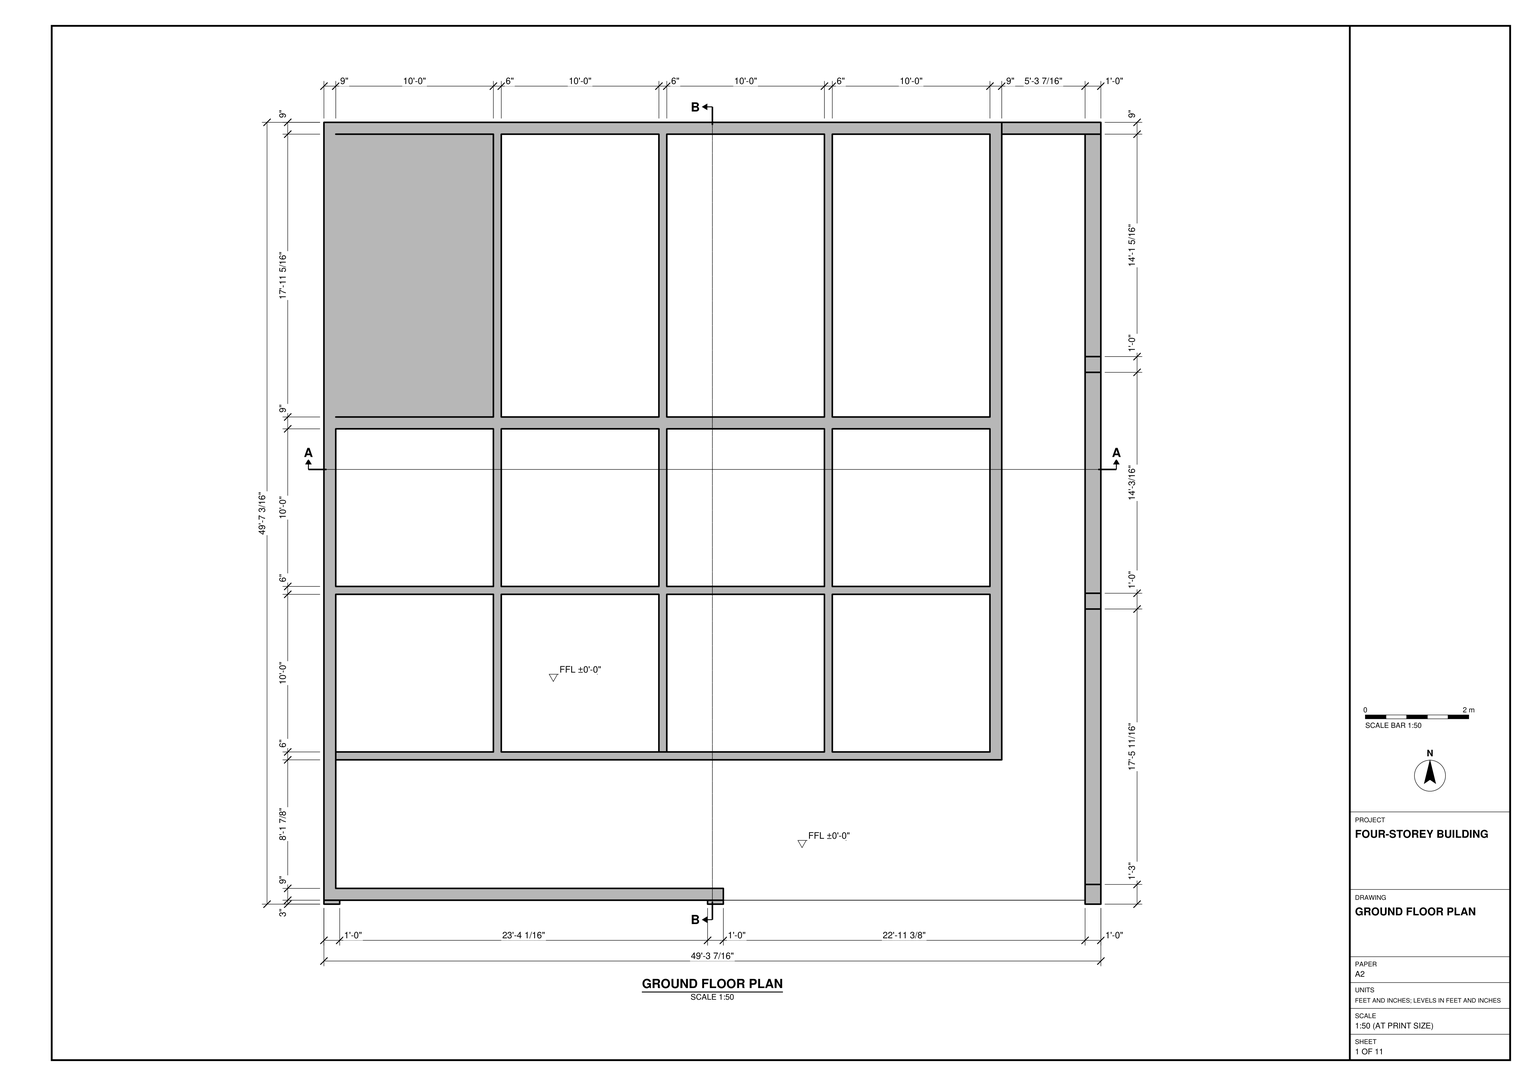
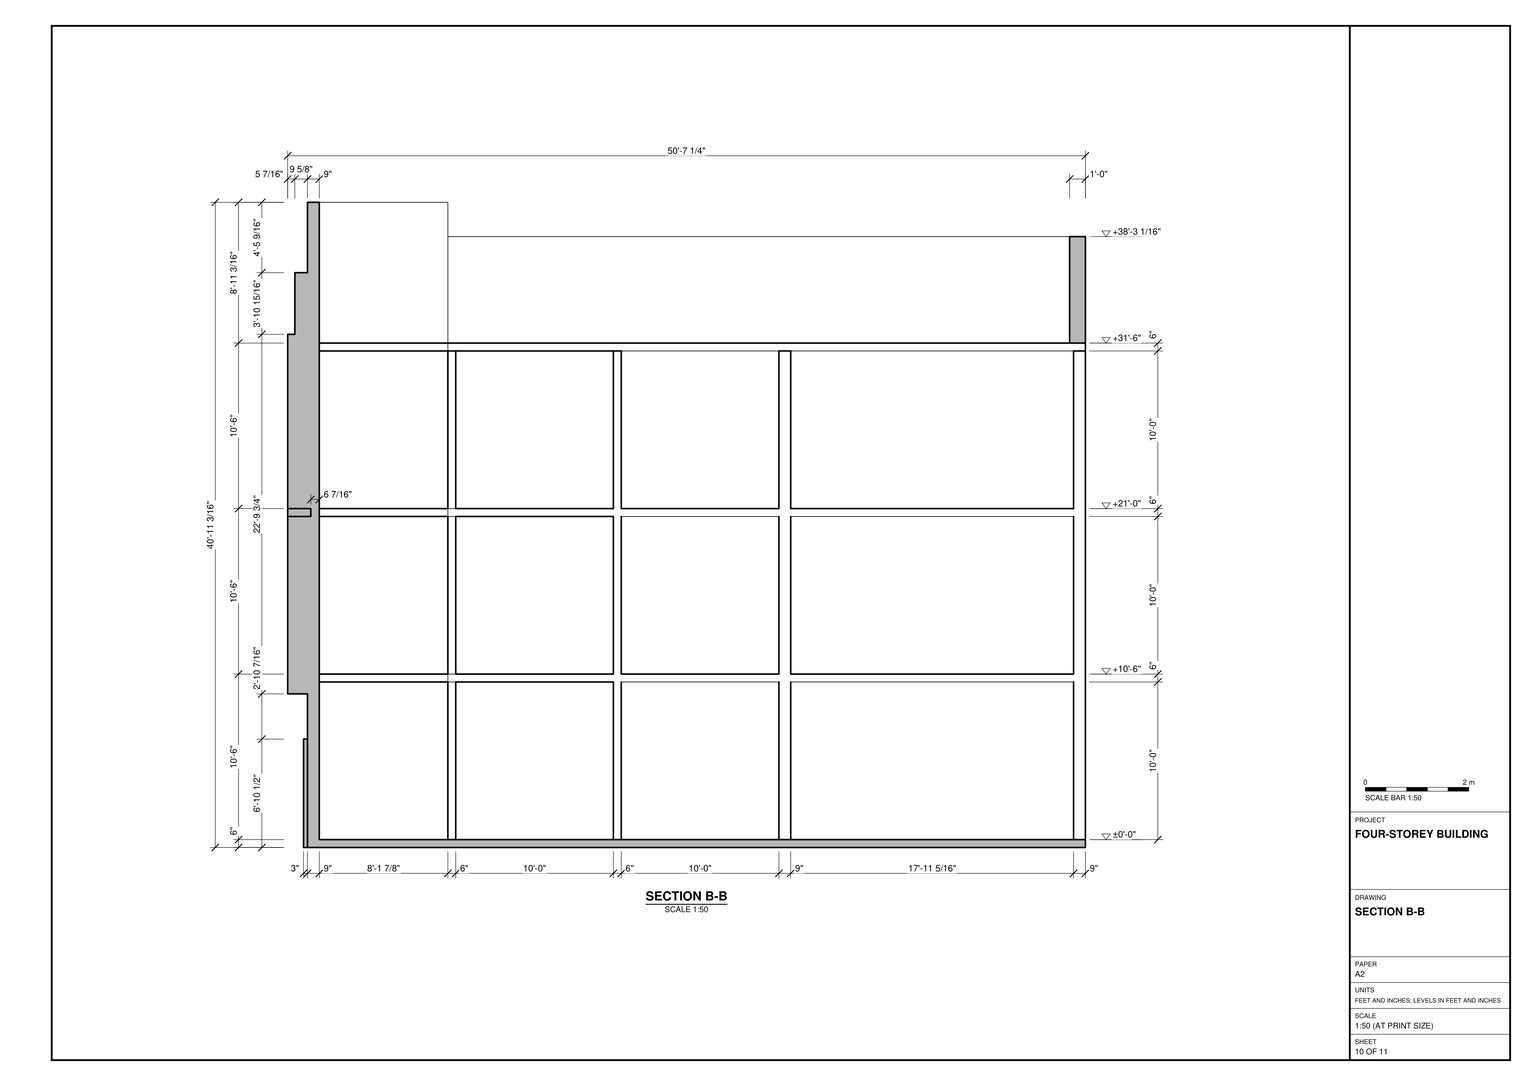
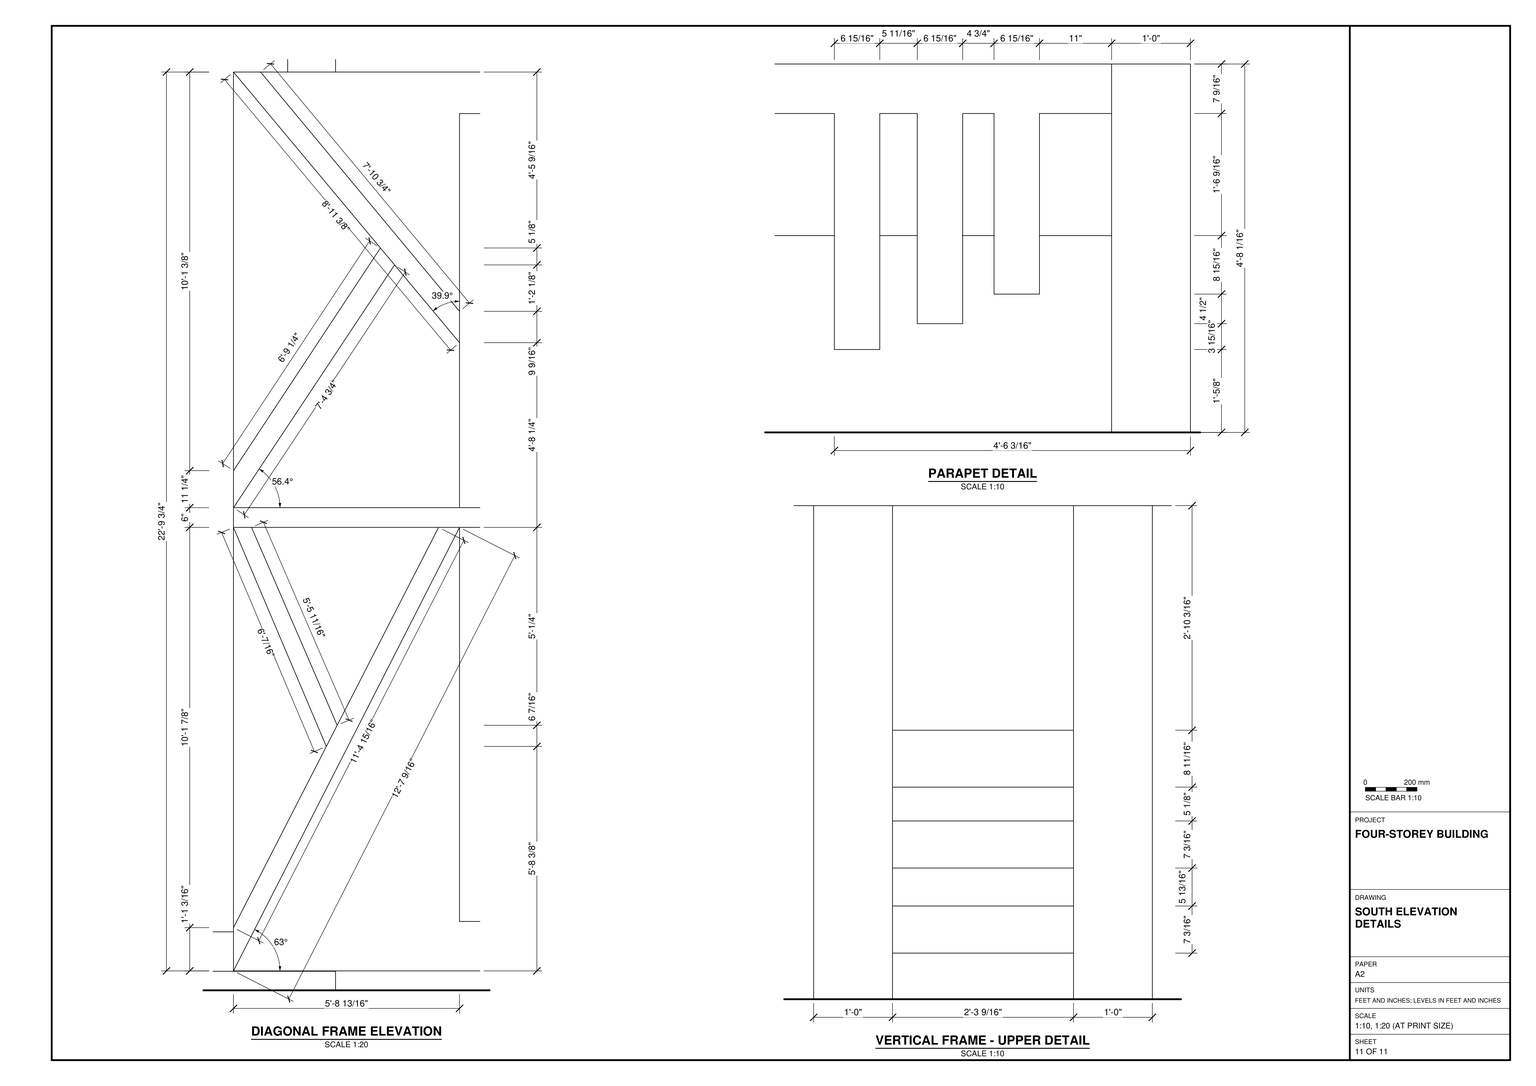
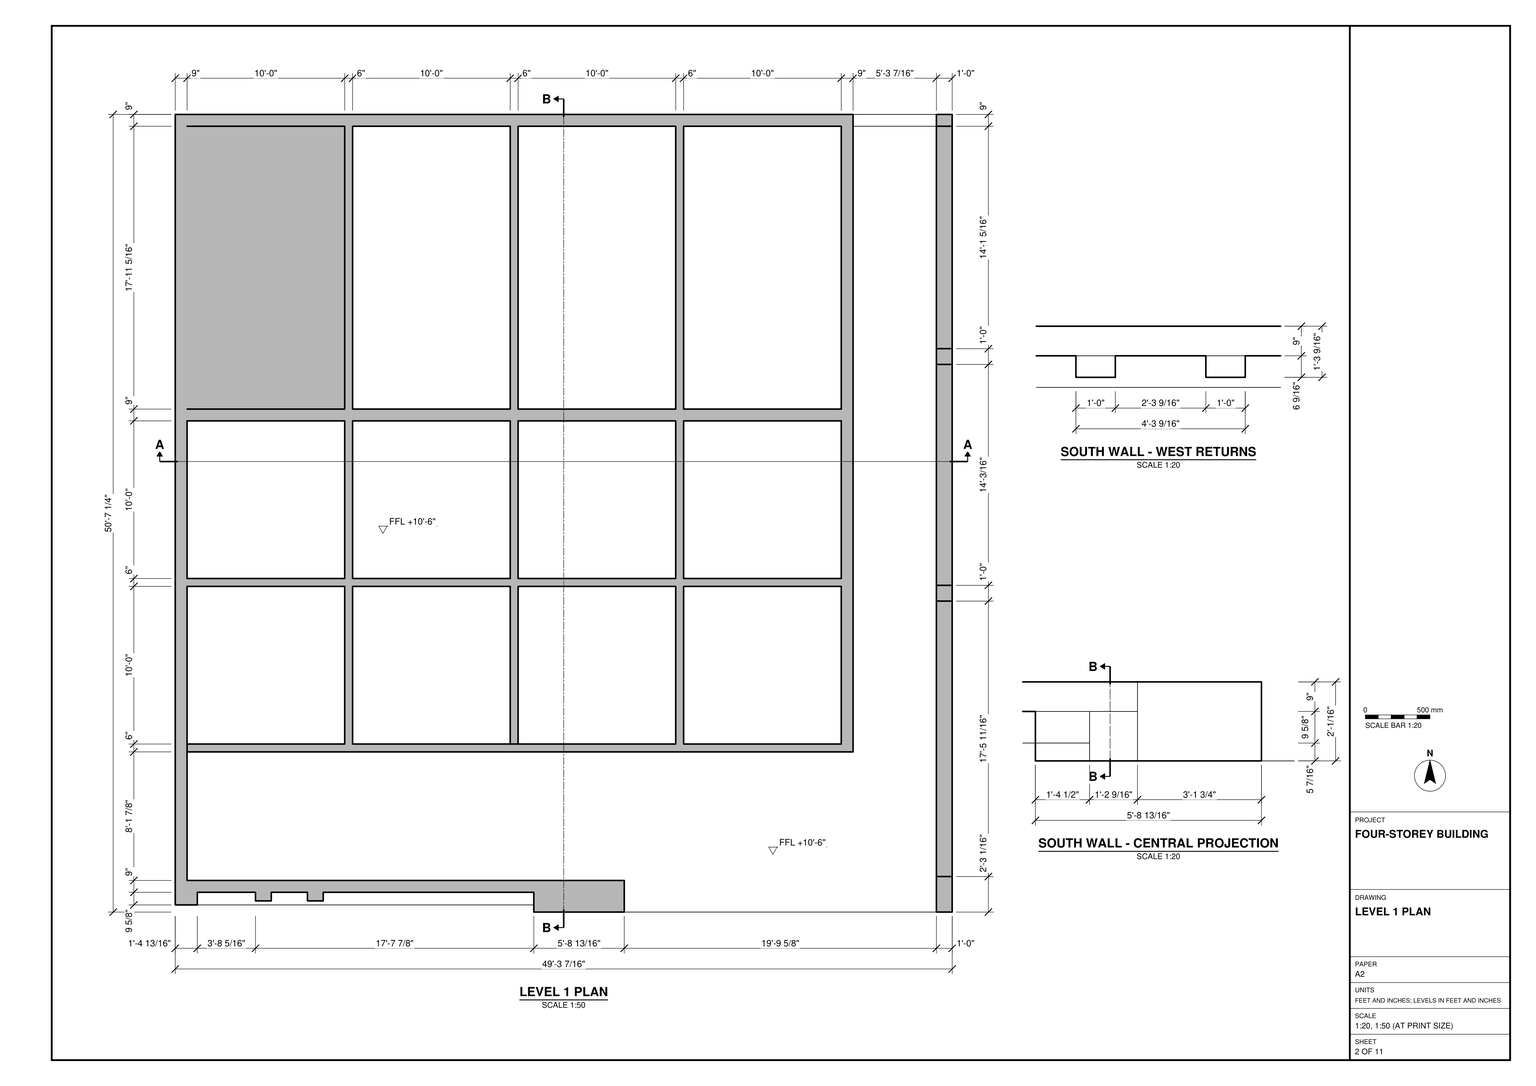
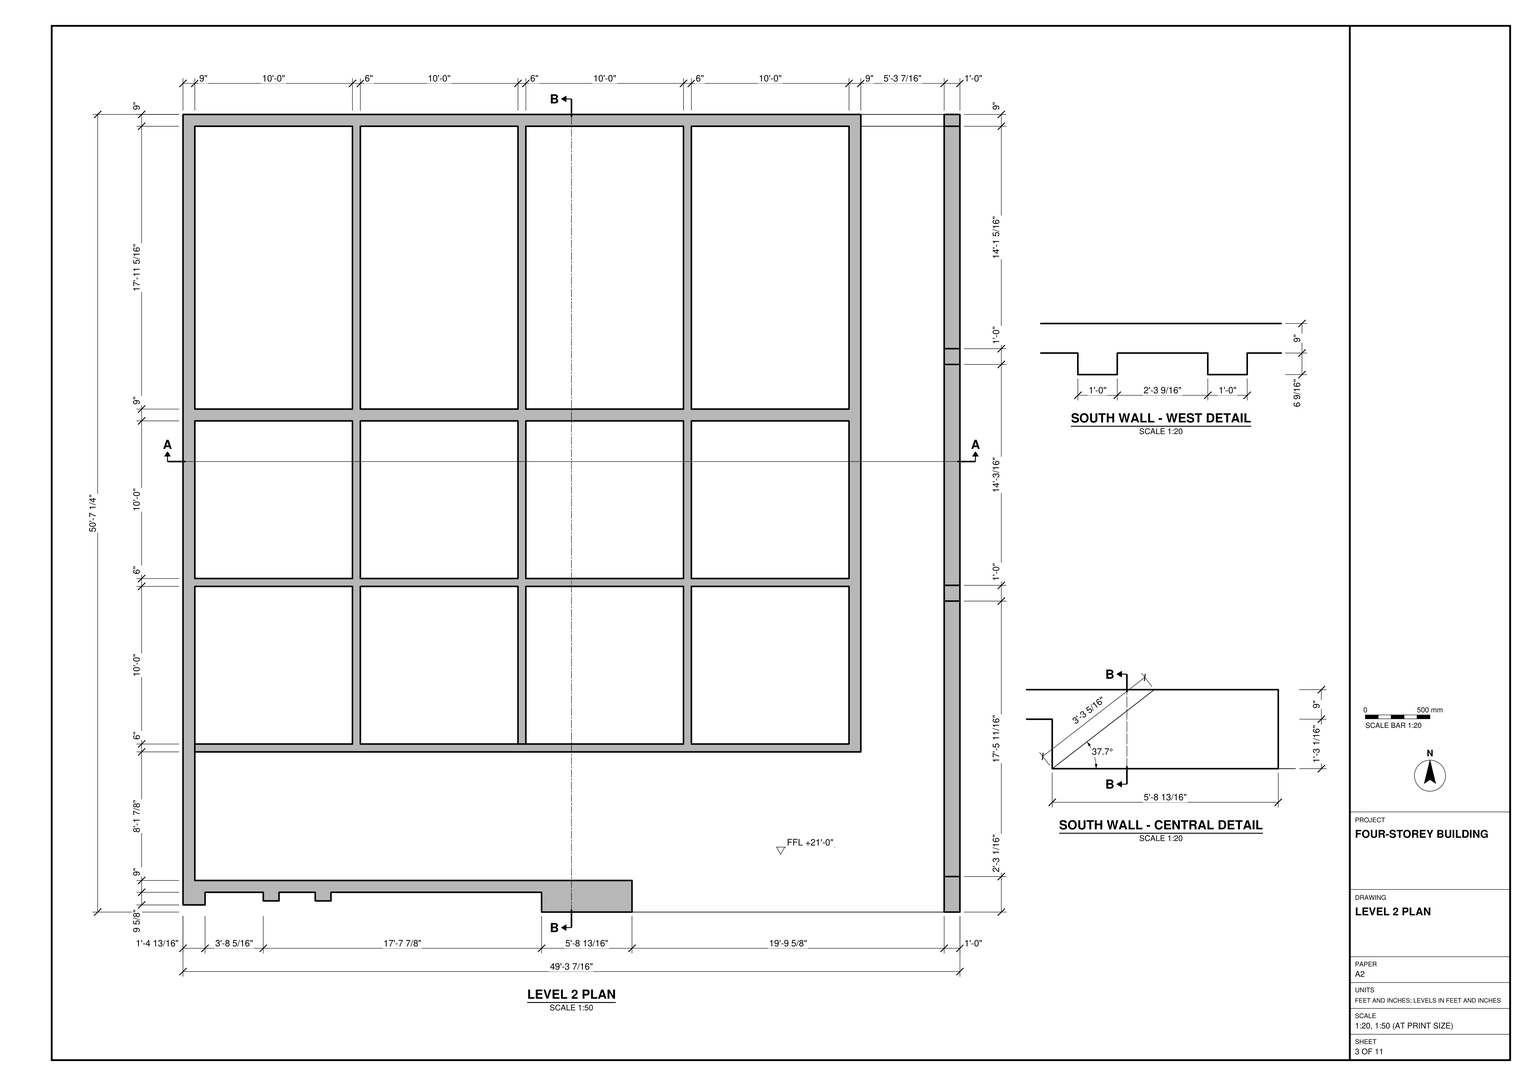
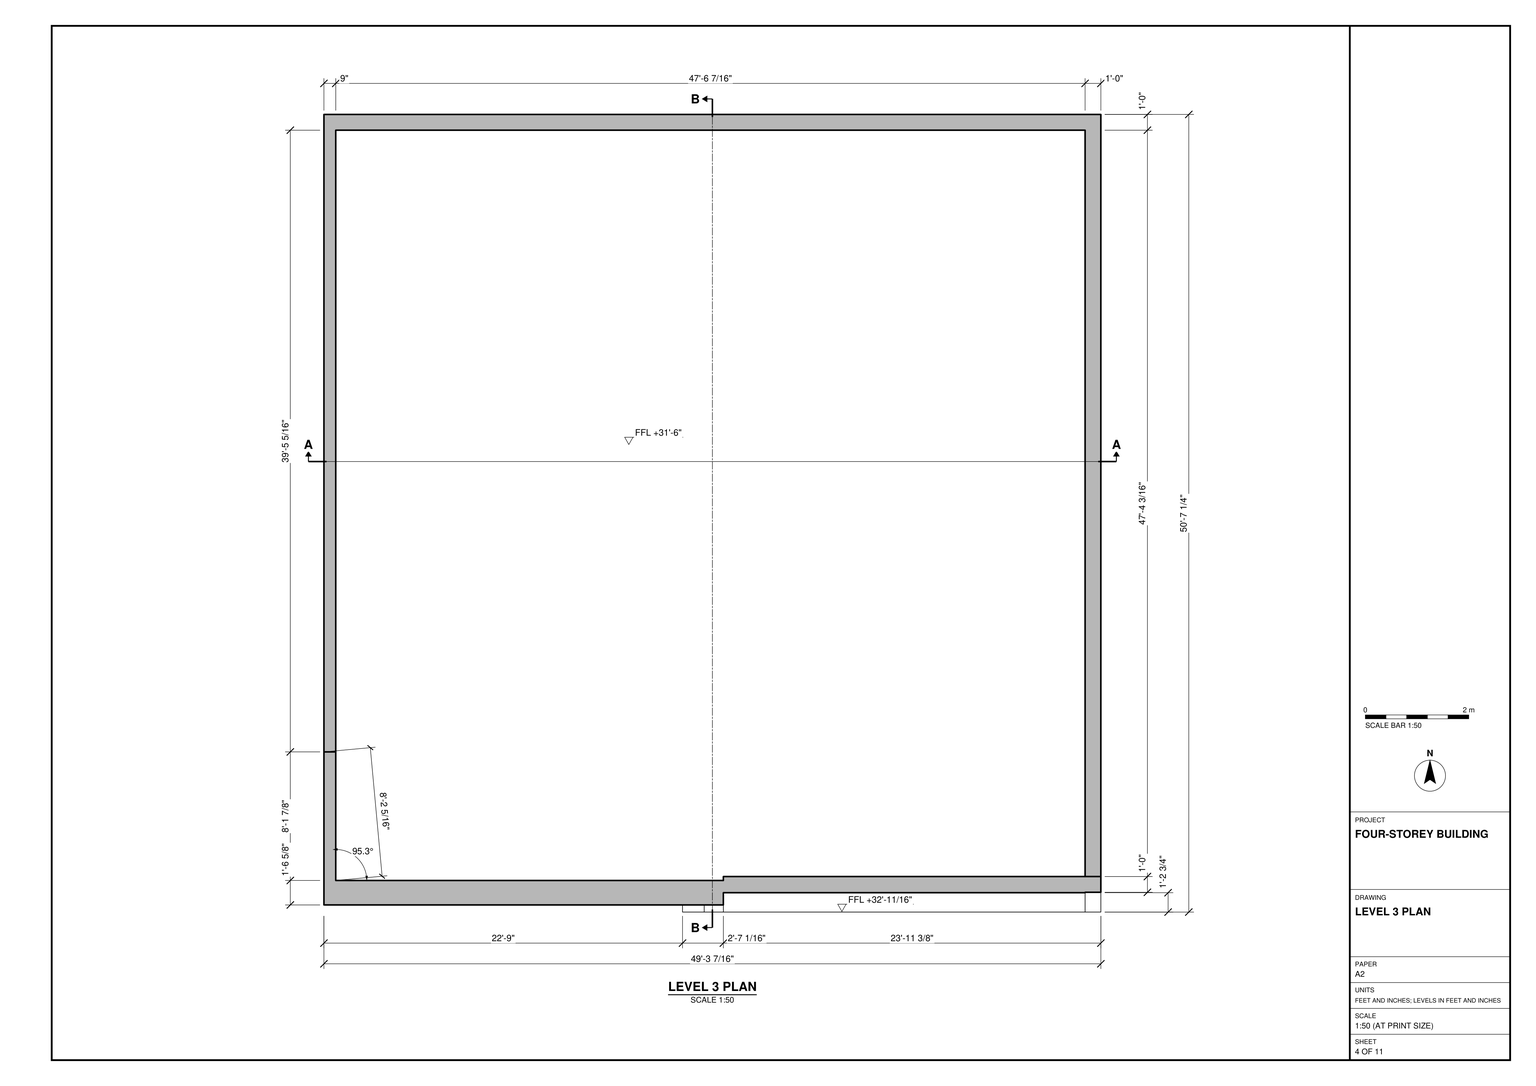
Build the four-storey building in SketchUp from task_files/diagram_01.pdf. Work in feet and inches. The overall extents, including the projecting elevation details, are 49'-3 7/16" along X, 50'-7 1/4" along Y and 40'-11 3/16" along Z. Set the floor levels at ±0'-0", +10'-6", +21'-0" and +31'-6".

Lay out the ground floor with four bays across the main block. Keep the deeper row of bays on the north side and the strips outside the grid on the east and south sides. Follow the wall thicknesses on each plan, distinguishing the 6" partitions from the 9" walls and the wider perimeter members. Use the sections to place the slabs, walls and flat roof relative to the floor levels. Follow the corresponding sheets for openings, stairs, built-in joinery and main furniture wherever shown. On the south elevation, model the stacked diagonal frames, the horizontal divisions between the vertical frame members and the stepped parapet detail. Use the section as well as the elevation to establish how far the facade projects.

Keep shell elements such as walls, slabs and roof in separate groups or components. Group each furniture or joinery piece separately and use components for repeated parts. Decor and loose items shown may be any suitable library components. Save one SketchUp model as output_files/four_storey_building_with_its_framed_south_elevation.skp.

# SketchUp Ruby script. Lengths in inches.
U = 1.inch
M = Sketchup.active_model
def pt(a) = Geom::Point3d.new(a.map { |v| v * U })
def face(e, loops, mat)
  f = e.add_face(loops[0].map { |a| pt(a) })
  loops[1..].each { |l| e.add_face(l.map { |a| pt(a) }).erase! }
  f.material = f.back_material = mat if mat
  f
end
# faces: each face lists its corners as indices into pts; further lists are holes
def faces(e, pts, list, mat = nil) = list.each { |f| face(e, (f[0].is_a?(Array) ? f : [f]).map { |l| l.map { |i| pts[i] } }, mat) }
# xy, xz, yz: faces in a plane at the given z, y or x. An outline is a flat list of corners, or four numbers for a rectangle; further outlines are holes
def ring(l) = l.size == 4 ? [[l[0], l[1]], [l[2], l[1]], [l[2], l[3]], [l[0], l[3]]] : l.each_slice(2).to_a
def flat(e, list, mat, &to3) = list.each { |f| face(e, (f[0].is_a?(Array) ? f : [f]).map { |l| ring(l).map { |u, v| to3.(u, v) } }, mat) }
def xy(e, z, list, mat = nil) = flat(e, list, mat) { |x, y| [x, y, z] }
def xz(e, y, list, mat = nil) = flat(e, list, mat) { |x, z| [x, y, z] }
def yz(e, x, list, mat = nil) = flat(e, list, mat) { |y, z| [x, y, z] }
def lines(e, pts, list) = list.each { |a, b| e.add_line(pt(pts[a]), pt(pts[b])) }
# prism: a flat outline (further loops are holes) pulled along v
def prism(e, loops, v, mat = nil)
  f = face(e, loops, mat); d = Geom::Vector3d.new(v.map { |x| x * U })
  f.pushpull(f.normal.samedirection?(d) ? d.length : -d.length)
end
def box(e, o, s, mat = nil) = prism(e, [[o, [o[0] + s[0], o[1], o[2]], [o[0] + s[0], o[1] + s[1], o[2]], [o[0], o[1] + s[1], o[2]]]], [0, 0, s[2]], mat)
def at(x, y, z, deg = 0) = Geom::Transformation.translation(pt([x, y, z])) * Geom::Transformation.rotation(ORIGIN, Z_AXIS, deg.degrees)
def axes(o, x, y, z) = Geom::Transformation.new([*x, 0, *y, 0, *z, 0, *pt(o).to_a, 1])
def part(name) = M.definitions.add(name)
# library, detail: a bought-in or finely detailed component or shape, given as its bounding box
def library(name, o, s) = part(name).tap { |d| box(d.entities, o, s) }
def detail(e, o, s) = box(e.add_group.entities, o, s)
def put(e, d, t, mat = nil) = e.add_instance(d, t).tap { |i| i.material = mat if mat }
def group(e, t, mat = nil) = e.add_group.tap { |g| g.transformation = t; g.material = mat if mat }.entities
root = M.entities
M.materials.add("[0007_MistyRose]").color = [137, 123, 121]
M.materials.add("[0008_LavenderBlush]").color = [168, 158, 161]
M.materials.add("[0012_Bisque]").color = [186, 166, 143]
M.materials.add("[0012_Bisque]1").color = [84, 74, 64]
M.materials.add("[0014_DarkSalmon]").color = [142, 91, 74]
M.materials.add("[0040_Peru]").color = [104, 67, 32]
M.materials.add("[0042_Sienna]").color = [76, 39, 21]
M.materials.add("[0111_SlateGray]").color = [53, 61, 68]
M.materials.add("[0118_Thistle]").color = [216, 191, 216]
M.materials.add("[Brick Tumbled]").color = [104, 102, 102]
M.materials.add("[Sketchy Stone]").color = [143, 143, 143]
M.materials.add("[Translucent Glass Gray]").color = [128, 128, 128]
M.materials["[Translucent Glass Gray]"].alpha = 0.5
xy(root,0,[[0,12.0625,12,15.0625],[579.4375,12.0625,579.4375,15.0625,0,15.0625,0,607.25,591.4375,607.25,591.4375,12.0625],[292.06,12.0625,304.06,15.0625]])
xy(root,6,[[304.06,15.0625,579.4375,15.0625,579.4375,598.25,516,598.25,516,121.9375,9,121.9375,9,24.0625,304.06,24.0625],[579.4375,27.0625,591.4375,236.75],[[0,121.9375,0,607.25,516,607.25,516,121.9375,387,121.9375,387,127.9375,507,127.9375,507,247.9375,387,247.9375,387,121.9375,381,121.9375,381,247.9375,261,247.9375,261,127.9375,255,127.9375,255,247.9375,135,247.9375,135,127.9375,381,127.9375,381,121.9375,9,121.9375,9,127.9375,129,127.9375,129,247.9375,9,247.9375,9,121.9375],[387,382.9375,507,598.25],[261,382.9375,381,598.25],[135,382.9375,255,598.25],[9,382.9375,129,598.25],[387,253.9375,507,373.9375],[9,253.9375,129,373.9375],[135,253.9375,255,373.9375],[261,253.9375,381,373.9375]],[9,127.9375,129,247.9375],[135,127.9375,255,247.9375],
  [261,127.9375,381,247.9375],[387,127.9375,507,247.9375],[579.4375,248.75,591.4375,416.92],[9,253.9375,129,373.9375],[135,253.9375,255,373.9375],
  [261,253.9375,381,373.9375],[387,253.9375,507,373.9375],[9,382.9375,129,598.25],[135,382.9375,255,598.25],[261,382.9375,381,598.25],
  [387,382.9375,507,598.25],[579.4375,416.92,591.4375,428.92],[579.4375,428.92,591.4375,598.25]])
xy(root,66,[[579.4375,27.0625,591.4375,236.75],[579.4375,248.75,591.4375,416.92],[579.4375,428.92,591.4375,598.25],[516,598.25,579.4375,607.25]])
xy(root,82.52,[[0,12.0625,12,15.0625],[292.06,12.0625,304.06,15.0625],[579.4375,12.0625,591.4375,15.0625]])
xy(root,116.83,[[0,5.4375,289.47,15.0625]])
xy(root,116.9375,[[272.97,0,289.47,5.4375],[289.47,0,304.06,15.0625],[304.06,0,579.4375,27.0625],[579.4375,0,591.4375,15.0625]])
xy(root,126,[[425.41,63.38,422.34,64.04,419.56,65.48,417.24,67.58,415.54,70.21,414.58,73.2,414.43,76.32,415.09,79.39,416.52,82.17,418.63,84.49,421.26,86.19,424.25,87.15,427.375,87.3,430.4375,86.64,433.22,85.21,435.54,83.1,437.24,80.47,438.2,77.49,438.35,74.36,437.6875,71.3,436.26,68.51,434.15,66.1875,431.52,64.49,428.54,63.53],[546.95,82.38,543.84,82.79,540.95,83.99,538.47,85.9,536.56,88.38,535.36,91.28,534.95,94.38,535.36,97.49,536.56,100.38,538.47,102.87,540.95,104.78,543.84,105.97,546.95,106.38,550.06,105.97,552.95,104.78,555.4375,102.87,557.34,100.38,558.54,97.49,558.95,94.38,558.54,91.28,557.34,88.38,555.4375,85.9,552.95,83.99,550.06,82.79],[546.95,330.38,543.84,330.79,540.95,331.99,538.47,333.9,536.56,336.38,535.36,339.28,534.95,342.38,535.36,345.49,536.56,348.38,538.47,350.87,540.95,352.78,543.84,353.97,546.95,354.38,550.06,353.97,552.95,352.78,555.4375,350.87,557.34,348.38,558.54,345.49,558.95,342.38,558.54,339.28,557.34,336.38,555.4375,333.9,552.95,331.99,550.06,330.79],[546.95,507.82,543.84,508.23,540.95,509.43,538.47,511.34,536.56,513.82,535.36,516.72,534.95,519.82,535.36,522.93,536.56,525.82,538.47,528.31,540.95,530.21,543.84,531.41,546.95,531.82,550.06,531.41,552.95,530.21,555.4375,528.31,557.34,525.82,558.54,522.93,558.95,519.82,558.54,516.72,557.34,513.82,555.4375,511.34,552.95,509.43,550.06,508.23]])
xy(root,126,[[[9,24.0625,9,247.9375,129,247.9375,129,127.9375,9,127.9375,9,121.9375,381,121.9375,381,127.9375,135,127.9375,135,247.9375,255,247.9375,255,127.9375,261,127.9375,261,247.9375,381,247.9375,381,121.9375,387,121.9375,387,247.9375,507,247.9375,507,127.9375,387,127.9375,387,121.9375,516,121.9375,516,607.25,591.4375,607.25,591.4375,27.0625,304.06,27.0625,304.06,24.0625],[425.41,63.38,428.54,63.53,431.52,64.49,434.15,66.1875,436.26,68.51,437.6875,71.3,438.35,74.36,438.2,77.49,437.24,80.47,435.54,83.1,433.22,85.21,430.4375,86.64,427.375,87.3,424.25,87.15,421.26,86.19,418.63,84.49,416.52,82.17,415.09,79.39,414.43,76.32,414.58,73.2,415.54,70.21,417.24,67.58,419.56,65.48,422.34,64.04],[546.95,507.82,550.06,508.23,552.95,509.43,555.4375,511.34,557.34,513.82,558.54,516.72,558.95,519.82,558.54,522.93,557.34,525.82,555.4375,528.31,552.95,530.21,550.06,531.41,546.95,531.82,543.84,531.41,540.95,530.21,538.47,528.31,536.56,525.82,535.36,522.93,534.95,519.82,535.36,516.72,536.56,513.82,538.47,511.34,540.95,509.43,543.84,508.23],[546.95,330.38,550.06,330.79,552.95,331.99,555.4375,333.9,557.34,336.38,558.54,339.28,558.95,342.38,558.54,345.49,557.34,348.38,555.4375,350.87,552.95,352.78,550.06,353.97,546.95,354.38,543.84,353.97,540.95,352.78,538.47,350.87,536.56,348.38,535.36,345.49,534.95,342.38,535.36,339.28,536.56,336.38,538.47,333.9,540.95,331.99,543.84,330.79],[546.95,82.38,550.06,82.79,552.95,83.99,555.4375,85.9,557.34,88.38,558.54,91.28,558.95,94.38,558.54,97.49,557.34,100.38,555.4375,102.87,552.95,104.78,550.06,105.97,546.95,106.38,543.84,105.97,540.95,104.78,538.47,102.87,536.56,100.38,535.36,97.49,534.95,94.38,535.36,91.28,536.56,88.38,538.47,85.9,540.95,83.99,543.84,82.79]]],"[0118_Thistle]")
xy(root,128.83,[[16.78,5.4375,272.97,5.4375,272.97,15.0625,112.66,15.0625,112.66,8.5,100.66,8.5,100.66,15.0625,73.1,15.0625,73.1,8.5,61.1,8.5,61.1,15.0625,16.78,15.0625]],"[0007_MistyRose]")
xy(root,132,[[341.81,0,579.4375,0,579.4375,598.25,516,598.25,516,121.9375,9,121.9375,9,24.0625,341.81,24.0625],[579.4375,27.0625,591.4375,236.75],[9,127.9375,129,247.9375],[135,127.9375,255,247.9375],[261,127.9375,381,247.9375],
  [387,127.9375,507,247.9375],[579.4375,236.75,591.4375,248.75],[579.4375,248.75,591.4375,416.92],[9,253.9375,129,373.9375],[135,253.9375,255,373.9375],
  [261,253.9375,381,373.9375],[387,253.9375,507,373.9375],[9,382.9375,129,598.25],[135,382.9375,255,598.25],[261,382.9375,381,598.25],
  [387,382.9375,507,598.25],[579.4375,416.92,591.4375,428.92],[579.4375,428.92,591.4375,598.25],[516,598.25,591.4375,607.25]])
xy(root,192,[[579.4375,27.0625,591.4375,236.75],[579.4375,248.75,591.4375,416.92],[579.4375,428.92,591.4375,598.25]])
xy(root,252,[[272.97,0,304.06,24.0625,341.81,24.0625,341.81,0],[436.4,56.91,433.3,57.3125,430.4,58.51,427.92,60.42,426.01,62.91,424.8125,65.8,424.4,68.91,424.8125,72.01,426.01,74.91,427.92,77.39,430.4,79.3,433.3,80.5,436.4,80.91,439.51,80.5,442.4,79.3,444.89,77.39,446.79,74.91,447.99,72.01,448.4,68.91,447.99,65.8,446.79,62.91,444.89,60.42,442.4,58.51,439.51,57.3125],[543.8,67.53,540.7,67.94,537.8,69.14,535.32,71.05,533.41,73.53,532.21,76.43,531.8,79.53,532.21,82.64,533.41,85.53,535.32,88.02,537.8,89.93,540.7,91.125,543.8,91.53,546.91,91.125,549.8,89.93,552.29,88.02,554.19,85.53,555.39,82.64,555.8,79.53,555.39,76.43,554.19,73.53,552.29,71.05,549.8,69.14,546.91,67.94],[552.8,315.85,549.7,316.25,546.8,317.45,544.32,319.36,542.41,321.85,541.21,324.74,540.8,327.85,541.21,330.95,542.41,333.85,544.32,336.33,546.8,338.24,549.7,339.4375,552.8,339.85,555.91,339.4375,558.8,338.24,561.29,336.33,563.19,333.85,564.39,330.95,564.8,327.85,564.39,324.74,563.19,321.85,561.29,319.36,558.8,317.45,555.91,316.25],[566.34,501.16,563.23,501.5625,560.34,502.76,557.85,504.67,555.95,507.16,554.75,510.05,554.34,513.16,554.75,516.26,555.95,519.16,557.85,521.64,560.34,523.55,563.23,524.75,566.34,525.16,569.45,524.75,572.34,523.55,574.82,521.64,576.73,519.16,577.93,516.26,578.34,513.16,577.93,510.05,576.73,507.16,574.82,504.67,572.34,502.76,569.45,501.5625]])
xy(root,252,[[[341.81,0,341.81,24.0625,9,24.0625,9,247.9375,129,247.9375,129,127.9375,9,127.9375,9,121.9375,381,121.9375,381,127.9375,135,127.9375,135,247.9375,255,247.9375,255,127.9375,261,127.9375,261,247.9375,381,247.9375,381,121.9375,387,121.9375,387,247.9375,507,247.9375,507,127.9375,387,127.9375,387,121.9375,516,121.9375,516,607.25,591.4375,607.25,591.4375,0],[552.8,315.85,555.91,316.25,558.8,317.45,561.29,319.36,563.19,321.85,564.39,324.74,564.8,327.85,564.39,330.95,563.19,333.85,561.29,336.33,558.8,338.24,555.91,339.4375,552.8,339.85,549.7,339.4375,546.8,338.24,544.32,336.33,542.41,333.85,541.21,330.95,540.8,327.85,541.21,324.74,542.41,321.85,544.32,319.36,546.8,317.45,549.7,316.25],[566.34,501.16,569.45,501.5625,572.34,502.76,574.82,504.67,576.73,507.16,577.93,510.05,578.34,513.16,577.93,516.26,576.73,519.16,574.82,521.64,572.34,523.55,569.45,524.75,566.34,525.16,563.23,524.75,560.34,523.55,557.85,521.64,555.95,519.16,554.75,516.26,554.34,513.16,554.75,510.05,555.95,507.16,557.85,504.67,560.34,502.76,563.23,501.5625],[436.4,56.91,439.51,57.3125,442.4,58.51,444.89,60.42,446.79,62.91,447.99,65.8,448.4,68.91,447.99,72.01,446.79,74.91,444.89,77.39,442.4,79.3,439.51,80.5,436.4,80.91,433.3,80.5,430.4,79.3,427.92,77.39,426.01,74.91,424.8125,72.01,424.4,68.91,424.8125,65.8,426.01,62.91,427.92,60.42,430.4,58.51,433.3,57.3125],[543.8,67.53,546.91,67.94,549.8,69.14,552.29,71.05,554.19,73.53,555.39,76.43,555.8,79.53,555.39,82.64,554.19,85.53,552.29,88.02,549.8,89.93,546.91,91.125,543.8,91.53,540.7,91.125,537.8,89.93,535.32,88.02,533.41,85.53,532.21,82.64,531.8,79.53,532.21,76.43,533.41,73.53,535.32,71.05,537.8,69.14,540.7,67.94]]],"[0118_Thistle]")
xy(root,258,[[341.81,0,579.4375,0,579.4375,598.25,516,598.25,516,121.9375,9,121.9375,9,24.0625,341.81,24.0625],[272.97,0,341.81,0,341.81,24.0625,304.06,24.0625],[579.4375,0,591.4375,27.0625],[579.4375,27.0625,591.4375,236.75],[9,127.9375,129,247.9375],
  [135,127.9375,255,247.9375],[261,127.9375,381,247.9375],[387,127.9375,507,247.9375],[579.4375,236.75,591.4375,248.75],[579.4375,248.75,591.4375,416.92],
  [9,253.9375,129,373.9375],[135,253.9375,255,373.9375],[261,253.9375,381,373.9375],[387,253.9375,507,373.9375],[9,382.9375,129,598.25],
  [135,382.9375,255,598.25],[261,382.9375,381,598.25],[387,382.9375,507,598.25],[579.4375,416.92,591.4375,428.92],[579.4375,428.92,591.4375,598.25],
  [516,598.25,591.4375,607.25]])
xy(root,318,[[579.4375,27.0625,591.4375,236.75],[579.4375,248.75,591.4375,416.92],[579.4375,428.92,591.4375,598.25]])
xy(root,347.58,[[73.1,5.5,100.66,8.5]])
xy(root,354.74,[[73.1,5.5,100.66,8.5]])
xy(root,360.53,[[73.1,5.5,100.66,8.5]])
xy(root,367.69,[[73.1,5.5,100.66,8.5]])
xy(root,372.84,[[73.1,5.5,100.66,8.5]])
xy(root,378,[[9,24.0625,0,121.9375,9,121.9375],[436.4,56.91,433.3,57.3125,430.4,58.51,427.92,60.42,426.01,62.91,424.8125,65.8,424.4,68.91,424.8125,72.01,426.01,74.91,427.92,77.39,430.4,79.3,433.3,80.5,436.4,80.91,439.51,80.5,442.4,79.3,444.89,77.39,446.79,74.91,447.99,72.01,448.4,68.91,447.99,65.8,446.79,62.91,444.89,60.42,442.4,58.51,439.51,57.3125],[554.34,56.91,551.23,57.3125,548.34,58.51,545.85,60.42,543.95,62.91,542.75,65.8,542.34,68.91,542.75,72.01,543.95,74.91,545.85,77.39,548.34,79.3,551.23,80.5,554.34,80.91,557.45,80.5,560.34,79.3,562.82,77.39,564.73,74.91,565.93,72.01,566.34,68.91,565.93,65.8,564.73,62.91,562.82,60.42,560.34,58.51,557.45,57.3125],[[0,121.9375,0,607.25,516,607.25,516,121.9375,387,121.9375,387,127.9375,507,127.9375,507,247.9375,387,247.9375,387,121.9375,381,121.9375,381,247.9375,261,247.9375,261,127.9375,255,127.9375,255,247.9375,135,247.9375,135,127.9375,381,127.9375,381,121.9375,9,121.9375,9,127.9375,129,127.9375,129,247.9375,9,247.9375,9,121.9375],[387,382.9375,507,598.25],[261,382.9375,381,598.25],[135,382.9375,255,598.25],[9,382.9375,129,598.25],[387,253.9375,507,373.9375],[9,253.9375,129,373.9375],[135,253.9375,255,373.9375],[261,253.9375,381,373.9375]],[554.34,171.47,551.23,171.875,548.34,173.08,545.85,174.98,543.95,177.47,542.75,180.36,542.34,183.47,542.75,186.57,543.95,189.47,545.85,191.95,548.34,193.86,551.23,195.06,554.34,195.47,557.45,195.06,560.34,193.86,562.82,191.95,564.73,189.47,565.93,186.57,566.34,183.47,565.93,180.36,564.73,177.47,562.82,174.98,560.34,173.08,557.45,171.875],
  [554.34,312.84,551.23,313.25,548.34,314.45,545.85,316.36,543.95,318.84,542.75,321.74,542.34,324.84,542.75,327.95,543.95,330.84,545.85,333.33,548.34,335.24,551.23,336.43,554.34,336.84,557.45,336.43,560.34,335.24,562.82,333.33,564.73,330.84,565.93,327.95,566.34,324.84,565.93,321.74,564.73,318.84,562.82,316.36,560.34,314.45,557.45,313.25],[554.34,512.78,551.23,513.1875,548.34,514.39,545.85,516.3,543.95,518.78,542.75,521.67,542.34,524.78,542.75,527.89,543.95,530.78,545.85,533.27,548.34,535.17,551.23,536.37,554.34,536.78,557.45,536.37,560.34,535.17,562.82,533.27,564.73,530.78,565.93,527.89,566.34,524.78,565.93,521.67,564.73,518.78,562.82,516.3,560.34,514.39,557.45,513.1875]])
xy(root,378,[[[341.81,0,341.81,24.0625,9,24.0625,9,247.9375,129,247.9375,129,127.9375,9,127.9375,9,121.9375,381,121.9375,381,127.9375,135,127.9375,135,247.9375,255,247.9375,255,127.9375,261,127.9375,261,247.9375,381,247.9375,381,121.9375,387,121.9375,387,247.9375,507,247.9375,507,127.9375,387,127.9375,387,121.9375,516,121.9375,516,607.25,579.4375,607.25,579.4375,598.25,591.4375,598.25,591.4375,428.92,579.4375,428.92,579.4375,416.92,591.4375,416.92,591.4375,248.75,579.4375,248.75,579.4375,236.75,591.4375,236.75,591.4375,27.0625,579.4375,27.0625,579.4375,0],[554.34,312.84,557.45,313.25,560.34,314.45,562.82,316.36,564.73,318.84,565.93,321.74,566.34,324.84,565.93,327.95,564.73,330.84,562.82,333.33,560.34,335.24,557.45,336.43,554.34,336.84,551.23,336.43,548.34,335.24,545.85,333.33,543.95,330.84,542.75,327.95,542.34,324.84,542.75,321.74,543.95,318.84,545.85,316.36,548.34,314.45,551.23,313.25],[554.34,512.78,557.45,513.1875,560.34,514.39,562.82,516.3,564.73,518.78,565.93,521.67,566.34,524.78,565.93,527.89,564.73,530.78,562.82,533.27,560.34,535.17,557.45,536.37,554.34,536.78,551.23,536.37,548.34,535.17,545.85,533.27,543.95,530.78,542.75,527.89,542.34,524.78,542.75,521.67,543.95,518.78,545.85,516.3,548.34,514.39,551.23,513.1875],[554.34,56.91,557.45,57.3125,560.34,58.51,562.82,60.42,564.73,62.91,565.93,65.8,566.34,68.91,565.93,72.01,564.73,74.91,562.82,77.39,560.34,79.3,557.45,80.5,554.34,80.91,551.23,80.5,548.34,79.3,545.85,77.39,543.95,74.91,542.75,72.01,542.34,68.91,542.75,65.8,543.95,62.91,545.85,60.42,548.34,58.51,551.23,57.3125],[436.4,56.91,439.51,57.3125,442.4,58.51,444.89,60.42,446.79,62.91,447.99,65.8,448.4,68.91,447.99,72.01,446.79,74.91,444.89,77.39,442.4,79.3,439.51,80.5,436.4,80.91,433.3,80.5,430.4,79.3,427.92,77.39,426.01,74.91,424.8125,72.01,424.4,68.91,424.8125,65.8,426.01,62.91,427.92,60.42,430.4,58.51,433.3,57.3125],[554.34,171.47,557.45,171.875,560.34,173.08,562.82,174.98,564.73,177.47,565.93,180.36,566.34,183.47,565.93,186.57,564.73,189.47,562.82,191.95,560.34,193.86,557.45,195.06,554.34,195.47,551.23,195.06,548.34,193.86,545.85,191.95,543.95,189.47,542.75,186.57,542.34,183.47,542.75,180.36,543.95,177.47,545.85,174.98,548.34,173.08,551.23,171.875]]],"[0118_Thistle]")
xy(root,381.5,[[73.1,5.5,100.66,8.5]])
xy(root,384,[[9,24.0625,304.06,24.0625,304.06,27.0625,579.4375,27.0625,579.4375,595.25,9,595.25],[579.4375,27.0625,579.4375,595.25,9,595.25,9,121.9375,0,121.9375,0,607.25,591.4375,607.25,591.4375,27.0625]])
xy(root,390.66,[[272.97,0,289.47,15.0625],[289.47,0,304.06,5.4375]])
xy(root,390.66,[[304.06,0,579.4375,14.75],[579.4375,0,591.4375,15.0625]],"[0111_SlateGray]")
xy(root,415.7,[[16.78,5.4375,16.78,15.0625,61.1,15.0625,61.1,8.5,73.1,8.5,73.1,15.0625,100.66,15.0625,100.66,8.5,112.66,8.5,112.66,15.0625,289.47,15.0625,289.47,5.4375]])
xy(root,435.09,[[304.06,14.75,579.4375,27.0625]],"[Translucent Glass Gray]")
xy(root,437.59,[[0,5.4375,304.06,15.0625]],"[0111_SlateGray]")
xy(root,447.72,[[537.22,15.0625,544.14,24.0625]])
xy(root,451.65,[[549.85,15.0625,556.76,24.0625]])
xy(root,456.15,[[561.54,15.0625,568.45,24.0625]])
xy(root,465.0625,[[579.4375,27.0625,591.4375,27.0625,591.4375,607.25,0,607.25,0,121.9375,9,121.9375,9,595.25,579.4375,595.25]])
xy(root,483.65,[[304.06,15.0625,537.22,24.0625],[544.14,15.0625,549.85,24.0625],[556.76,15.0625,561.54,24.0625],[568.45,15.0625,579.4375,24.0625]])
xy(root,491.1875,[[0,15.0625,304.06,15.0625,304.06,24.0625,9,24.0625,9,121.9375,0,121.9375],[304.06,15.0625,579.4375,24.0625],[579.4375,15.0625,591.4375,27.0625]])
xz(root,0,[[272.97,116.9375,341.81,252,335.43,252,304.55,191.74,301.25,185.29,272.97,130.1],[301.25,185.29,304.55,191.74,278.47,252,272.97,252],[272.97,258,322.02,331.93,317.72,337.07,272.97,269.27],[341.81,308.24,341.81,317.79,281.22,390.66,272.97,390.66,317.72,337.07,322.02,331.93]],"[0007_MistyRose]")
xz(root,0,[[272.97,116.9375,591.4375,116.9375,591.4375,252,579.4375,252,579.4375,132,341.81,132,341.81,252],[272.97,130.1,301.25,185.29,272.97,252],[304.55,191.74,335.43,252,278.47,252],[272.97,252,591.4375,258],[272.97,258,341.81,258,341.81,308.24,322.02,331.93],
  [579.4375,258,591.4375,258,591.4375,390.66,281.22,390.66,341.81,317.79,341.81,378,579.4375,378],[272.97,269.27,317.72,337.07,272.97,390.66]],"[Sketchy Stone]")
xz(root,5.4375,[[0,116.83,289.47,116.83,289.47,116.9375,272.97,116.9375,272.97,128.83,16.78,128.83,16.78,415.7,289.47,415.7,289.47,390.66,304.06,390.66,304.06,437.59,0,437.59]],"[0008_LavenderBlush]")
xz(root,5.5,[[73.1,347.58,100.66,354.74],[73.1,360.53,100.66,367.69],[73.1,372.84,100.66,381.5]],"[0007_MistyRose]")
xz(root,8.5,[[73.1,347.58,100.66,354.74],[73.1,360.53,100.66,367.69],[73.1,372.84,100.66,381.5]])
xz(root,8.5,[[61.1,128.83,73.1,415.7],[100.66,128.83,112.66,415.7]],"[0007_MistyRose]")
xz(root,12.0625,[[0,0,12,82.52],[292.06,0,304.06,82.52],[579.4375,0,591.4375,82.52]],"[0014_DarkSalmon]")
xz(root,14.75,[[304.06,390.66,579.4375,435.09]],"[Translucent Glass Gray]")
xz(root,15.0625,[[0,0,12,82.52],[292.06,0,304.06,82.52],[579.4375,82.52,591.4375,116.9375],[289.47,116.83,304.06,116.9375]])
xz(root,15.0625,[[579.4375,390.66,591.4375,491.1875],[0,437.59,304.06,491.1875],[537.22,447.72,544.14,447.72,544.14,483.65,549.85,483.65,549.85,451.65,556.76,451.65,556.76,483.65,561.54,483.65,561.54,456.15,568.45,456.15,568.45,483.65,579.4375,483.65,579.4375,491.1875,304.06,491.1875,304.06,483.65,537.22,483.65]],"[0007_MistyRose]")
xz(root,15.0625,[[12,0,292.06,0,292.06,82.52,304.06,82.52,304.06,116.83,0,116.83,0,82.52,12,82.52]],"[0012_Bisque]")
xz(root,15.0625,[[304.06,0,579.4375,6]],"[0014_DarkSalmon]")
xz(root,15.0625,[[16.78,128.83,61.1,415.7],[73.1,128.83,100.66,415.7],[112.66,128.83,272.97,128.83,272.97,390.66,289.47,390.66,289.47,415.7,112.66,415.7]],"[Brick Tumbled]")
xz(root,24.0625,[[9,6,304.06,126],[9,126,304.06,132],[9,132,341.81,252],[9,252,304.06,258],[9,258,341.81,378],
  [9,378,304.06,384],[9,384,9,491.1875,579.4375,491.1875,579.4375,483.65,568.45,483.65,568.45,456.15,561.54,456.15,561.54,483.65,556.76,483.65,556.76,451.65,549.85,451.65,549.85,483.65,544.14,483.65,544.14,447.72,537.22,447.72,537.22,483.65,304.06,483.65,304.06,384]])
xz(root,27.0625,[[579.4375,6,591.4375,66],[579.4375,66,591.4375,126],[304.06,116.9375,579.4375,126],[579.4375,126,591.4375,132],[579.4375,132,591.4375,192],
  [579.4375,192,591.4375,258],[579.4375,258,591.4375,318],[579.4375,318,591.4375,378],[579.4375,384,591.4375,465.0625],[579.4375,465.0625,591.4375,491.1875]])
xz(root,27.0625,[[304.06,384,579.4375,435.09]],"[Translucent Glass Gray]")
xz(root,121.9375,[[0,378,9,384],[0,384,9,465.0625],[0,465.0625,9,491.1875]])
xz(root,121.9375,[[9,6,355.03,6,355.03,91.25,412.78,91.25,412.78,6,516,6,516,126,9,126],[9,132,355.03,132,355.03,217.25,412.78,217.25,412.78,132,516,132,516,252,9,252],[9,258,355.03,258,355.03,343.25,412.78,343.25,412.78,258,516,258,516,378,9,378]],"[0012_Bisque]")
xz(root,121.9375,[[355.03,6,412.78,91.25],[355.03,132,412.78,217.25],[355.03,258,412.78,343.25]],"[0042_Sienna]")
xz(root,127.9375,[[9,6,129,126],[135,6,255,126],[255,6,261,126],[261,6,381,126],[387,6,507,126],
  [9,132,129,252],[135,132,255,252],[255,132,261,252],[261,132,381,252],[387,132,507,252],
  [9,258,129,378],[135,258,255,378],[255,258,261,378],[261,258,381,378],[387,258,507,378]])
xz(root,236.75,[[579.4375,6,591.4375,66],[579.4375,66,591.4375,132],[579.4375,132,591.4375,192],[579.4375,192,591.4375,258],[579.4375,258,591.4375,318],
  [579.4375,318,591.4375,378]])
xz(root,247.9375,[[9,6,129,126],[135,6,255,126],[261,6,381,126],[387,6,507,126],[9,132,129,252],
  [135,132,255,252],[261,132,381,252],[387,132,507,252],[9,258,129,378],[135,258,255,378],
  [261,258,381,378],[387,258,507,378]])
xz(root,248.75,[[579.4375,6,591.4375,66],[579.4375,66,591.4375,132],[579.4375,132,591.4375,192],[579.4375,192,591.4375,258],[579.4375,258,591.4375,318],
  [579.4375,318,591.4375,378]])
xz(root,253.9375,[[9,6,129,126],[135,6,255,126],[261,6,381,126],[387,6,507,126],[9,132,129,252],
  [135,132,255,252],[261,132,381,252],[387,132,507,252],[9,258,129,378],[135,258,255,378],
  [261,258,381,378],[387,258,507,378]])
xz(root,373.9375,[[9,6,129,126],[135,6,255,126],[261,6,381,126],[387,6,507,126],[9,132,129,252],
  [135,132,255,252],[261,132,381,252],[387,132,507,252],[9,258,129,378],[135,258,255,378],
  [261,258,381,378],[387,258,507,378]])
xz(root,382.9375,[[9,6,129,126],[135,6,255,126],[261,6,381,126],[387,6,507,126],[9,132,129,252],
  [135,132,255,252],[261,132,381,252],[387,132,507,252],[9,258,129,378],[135,258,255,378],
  [261,258,381,378],[387,258,507,378]])
xz(root,416.92,[[579.4375,6,591.4375,66],[579.4375,66,591.4375,132],[579.4375,132,591.4375,192],[579.4375,192,591.4375,258],[579.4375,258,591.4375,318],
  [579.4375,318,591.4375,378]])
xz(root,428.92,[[579.4375,6,591.4375,66],[579.4375,66,591.4375,132],[579.4375,132,591.4375,192],[579.4375,192,591.4375,258],[579.4375,258,591.4375,318],
  [579.4375,318,591.4375,378]])
xz(root,595.25,[[9,384,579.4375,465.0625]])
xz(root,598.25,[[9,6,129,126],[135,6,255,126],[261,6,381,126],[387,6,507,126],[516,6,579.4375,66],
  [579.4375,6,591.4375,66],[579.4375,66,591.4375,132],[9,132,129,252],[135,132,255,252],[261,132,381,252],
  [387,132,507,252],[579.4375,132,591.4375,192],[579.4375,192,591.4375,258],[9,258,129,378],[135,258,255,378],
  [261,258,381,378],[387,258,507,378],[579.4375,258,591.4375,318],[579.4375,318,591.4375,378]])
xz(root,607.25,[[0,0,0,6,516,6,516,66,579.4375,66,579.4375,126,591.4375,126,591.4375,0],[0,6,516,126],[0,126,579.4375,132],[579.4375,126,591.4375,132],[0,132,516,252],
  [579.4375,132,591.4375,252],[0,252,579.4375,258],[579.4375,252,591.4375,258],[0,258,516,378],[579.4375,258,591.4375,378],
  [0,378,591.4375,384],[0,384,591.4375,465.0625]])
yz(root,0,[[12.0625,0,15.0625,6],[15.0625,0,607.25,6],[15.0625,6,15.0625,116.83,5.4375,116.83,5.4375,378,607.25,378,607.25,6],[12.0625,6,15.0625,82.52],[5.4375,378,121.9375,384],
  [121.9375,378,607.25,384],[5.4375,384,5.4375,437.59,15.0625,437.59,15.0625,491.1875,121.9375,491.1875,121.9375,384],[121.9375,384,607.25,465.0625]])
yz(root,9,[[24.0625,6,121.9375,126],[121.9375,6,127.9375,126],[127.9375,6,247.9375,126],[253.9375,6,373.9375,126],[24.0625,126,121.9375,132],
  [24.0625,132,121.9375,252],[121.9375,132,127.9375,252],[127.9375,132,247.9375,252],[253.9375,132,373.9375,252],[24.0625,252,121.9375,258],
  [24.0625,258,121.9375,378],[121.9375,258,127.9375,378],[127.9375,258,247.9375,378],[253.9375,258,373.9375,378],[382.9375,258,598.25,378],
  [24.0625,378,121.9375,384],[24.0625,384,121.9375,491.1875],[121.9375,384,595.25,465.0625]])
yz(root,12,[[12.0625,0,15.0625,82.52]],"[0040_Peru]")
yz(root,16.78,[[5.4375,128.83,15.0625,415.7]],"[0111_SlateGray]")
yz(root,61.1,[[8.5,128.83,15.0625,415.7]],"[0012_Bisque]1")
yz(root,73.1,[[5.5,347.58,8.5,354.74],[5.5,360.53,8.5,367.69],[5.5,372.84,8.5,381.5]])
yz(root,73.1,[[8.5,128.83,15.0625,415.7]],"[0007_MistyRose]")
yz(root,100.66,[[5.5,347.58,8.5,354.74],[5.5,360.53,8.5,367.69],[5.5,372.84,8.5,381.5]])
yz(root,100.66,[[8.5,128.83,15.0625,415.7]],"[0007_MistyRose]")
yz(root,112.66,[[8.5,128.83,15.0625,415.7]],"[0007_MistyRose]")
yz(root,129,[[127.9375,6,247.9375,126],[253.9375,6,373.9375,126],[382.9375,6,598.25,126],[127.9375,132,247.9375,252],[253.9375,132,373.9375,252],
  [382.9375,132,598.25,252],[127.9375,258,247.9375,378],[253.9375,258,373.9375,378],[382.9375,258,598.25,378]])
yz(root,135,[[127.9375,6,247.9375,126],[253.9375,6,373.9375,126],[382.9375,6,598.25,126],[127.9375,132,247.9375,252],[253.9375,132,373.9375,252],
  [382.9375,132,598.25,252],[127.9375,258,247.9375,378],[253.9375,258,373.9375,378],[382.9375,258,598.25,378]])
yz(root,255,[[127.9375,6,247.9375,126],[253.9375,6,373.9375,126],[382.9375,6,598.25,126],[127.9375,132,247.9375,252],[253.9375,132,373.9375,252],
  [382.9375,132,598.25,252],[127.9375,258,247.9375,378],[253.9375,258,373.9375,378],[382.9375,258,598.25,378]])
yz(root,261,[[127.9375,6,247.9375,126],[253.9375,6,373.9375,126],[382.9375,6,598.25,126],[127.9375,132,247.9375,252],[253.9375,132,373.9375,252],
  [382.9375,132,598.25,252],[127.9375,258,247.9375,378],[253.9375,258,373.9375,378],[382.9375,258,598.25,378]])
yz(root,272.97,[[0,116.9375,5.4375,128.83]])
yz(root,272.97,[[0,128.83,15.0625,390.66]],"[0007_MistyRose]")
yz(root,289.47,[[5.4375,116.83,15.0625,116.9375],[5.4375,390.66,15.0625,415.7]])
yz(root,292.06,[[12.0625,0,15.0625,82.52]])
yz(root,304.06,[[15.0625,6,24.0625,116.9375],[24.0625,116.9375,27.0625,126],[24.0625,384,27.0625,435.09]])
yz(root,304.06,[[12.0625,0,15.0625,6],[12.0625,6,15.0625,82.52]],"[0040_Peru]")
yz(root,304.06,[[5.4375,390.66,14.75,390.66,14.75,435.09,24.0625,435.09,24.0625,483.65,15.0625,483.65,15.0625,437.59,5.4375,437.59]],"[0111_SlateGray]")
yz(root,341.81,[[0,132,24.0625,252],[0,258,24.0625,378]],"[0012_Bisque]1")
yz(root,381,[[127.9375,6,247.9375,126],[253.9375,6,373.9375,126],[382.9375,6,598.25,126],[127.9375,132,247.9375,252],[253.9375,132,373.9375,252],
  [382.9375,132,598.25,252],[127.9375,258,247.9375,378],[253.9375,258,373.9375,378],[382.9375,258,598.25,378]])
yz(root,387,[[127.9375,6,247.9375,126],[253.9375,6,373.9375,126],[382.9375,6,598.25,126],[127.9375,132,247.9375,252],[253.9375,132,373.9375,252],
  [382.9375,132,598.25,252],[127.9375,258,247.9375,378],[253.9375,258,373.9375,378],[382.9375,258,598.25,378]])
yz(root,507,[[127.9375,6,247.9375,126],[253.9375,6,373.9375,126],[382.9375,6,598.25,126],[127.9375,132,247.9375,252],[253.9375,132,373.9375,252],
  [382.9375,132,598.25,252],[127.9375,258,247.9375,378],[253.9375,258,373.9375,378],[382.9375,258,598.25,378]])
yz(root,516,[[598.25,6,607.25,66],[598.25,66,607.25,126],[598.25,132,607.25,252],[598.25,258,607.25,378]])
yz(root,516,[[121.9375,6,598.25,126],[121.9375,132,598.25,252],[121.9375,258,598.25,378]],"[0012_Bisque]")
yz(root,537.22,[[15.0625,447.72,24.0625,483.65]])
yz(root,544.14,[[15.0625,447.72,24.0625,483.65]],"[0111_SlateGray]")
yz(root,549.85,[[15.0625,451.65,24.0625,483.65]])
yz(root,556.76,[[15.0625,451.65,24.0625,483.65]],"[0111_SlateGray]")
yz(root,561.54,[[15.0625,456.15,24.0625,483.65]])
yz(root,568.45,[[15.0625,456.15,24.0625,483.65]],"[0111_SlateGray]")
yz(root,579.4375,[[12.0625,0,15.0625,6],[12.0625,6,12.0625,82.52,15.0625,82.52,15.0625,116.9375,27.0625,116.9375,27.0625,6],[27.0625,6,236.75,66],[236.75,6,248.75,132],[248.75,6,416.92,66],
  [416.92,6,428.92,132],[428.92,6,598.25,66],[598.25,66,607.25,378],[0,132,27.0625,252],[27.0625,132,236.75,192],
  [236.75,132,248.75,258],[248.75,132,416.92,192],[416.92,132,428.92,258],[428.92,132,598.25,192],[0,258,27.0625,378],
  [27.0625,258,236.75,318],[236.75,258,248.75,378],[248.75,258,416.92,318],[416.92,258,428.92,378],[428.92,258,598.25,318],
  [27.0625,384,595.25,465.0625],[14.75,390.66,15.0625,435.09],[15.0625,435.09,15.0625,483.65,24.0625,483.65,24.0625,491.1875,27.0625,491.1875,27.0625,435.09]])
yz(root,591.4375,[[12.0625,0,607.25,0,607.25,126,598.25,126,598.25,6,248.75,6,248.75,66,236.75,66,236.75,6,12.0625,6],[27.0625,6,236.75,66],[248.75,6,416.92,66],[416.92,6,428.92,66],[428.92,6,598.25,66],
  [236.75,66,248.75,126],[416.92,66,428.92,126],[27.0625,126,236.75,132],[236.75,126,248.75,132],[248.75,126,416.92,132],
  [416.92,126,428.92,132],[428.92,126,598.25,132],[598.25,126,607.25,132],[27.0625,132,236.75,192],[236.75,132,248.75,192],
  [248.75,132,416.92,192],[416.92,132,428.92,192],[428.92,132,598.25,192],[598.25,132,607.25,252],[236.75,192,248.75,252],
  [416.92,192,428.92,252],[27.0625,252,236.75,258],[236.75,252,248.75,258],[248.75,252,416.92,258],[416.92,252,428.92,258],
  [428.92,252,598.25,258],[598.25,252,607.25,258],[27.0625,258,236.75,318],[236.75,258,248.75,318],[248.75,258,416.92,318],
  [416.92,258,428.92,318],[428.92,258,598.25,318],[598.25,258,607.25,378],[236.75,318,248.75,378],[416.92,318,428.92,378],
  [0,378,607.25,384],[27.0625,384,607.25,465.0625]])
yz(root,591.4375,[[12.0625,6,27.0625,6,27.0625,132,0,132,0,116.9375,15.0625,116.9375,15.0625,82.52,12.0625,82.52],[0,132,27.0625,252],[0,252,27.0625,258],[0,258,27.0625,378]],"[0012_Bisque]1")
yz(root,591.4375,[[0,384,27.0625,384,27.0625,491.1875,15.0625,491.1875,15.0625,390.66,0,390.66]],"[0111_SlateGray]")
p = [[272.97,0,258],[272.97,0,252],[304.06,24.0625,252],[304.06,24.0625,258],[381,127.9375,132],[381,121.9375,132],
  [9,121.9375,252],[0,121.9375,252],[387,127.9375,132],[387,121.9375,132],[381,127.9375,258],[381,121.9375,258],
  [387,127.9375,258],[387,121.9375,258],[9,24.0625,126],[0,24.0625,126],[9,24.0625,252],[0,24.0625,252],
  [304.06,15.0625,384],[304.06,24.0625,384],[579.4375,15.0625,384],[579.4375,27.0625,384],[12.875,607.25,396],[9,607.25,396],
  [579.4375,14.75,390.66],[587.81,14.75,390.66]]
faces(root,p,[[0,1,2,3]])
lines(root,p,[[4,5],[6,7],[8,9],[10,11],[12,13],[14,15],[16,17],[18,19],[20,21],[22,23],[24,25]])
